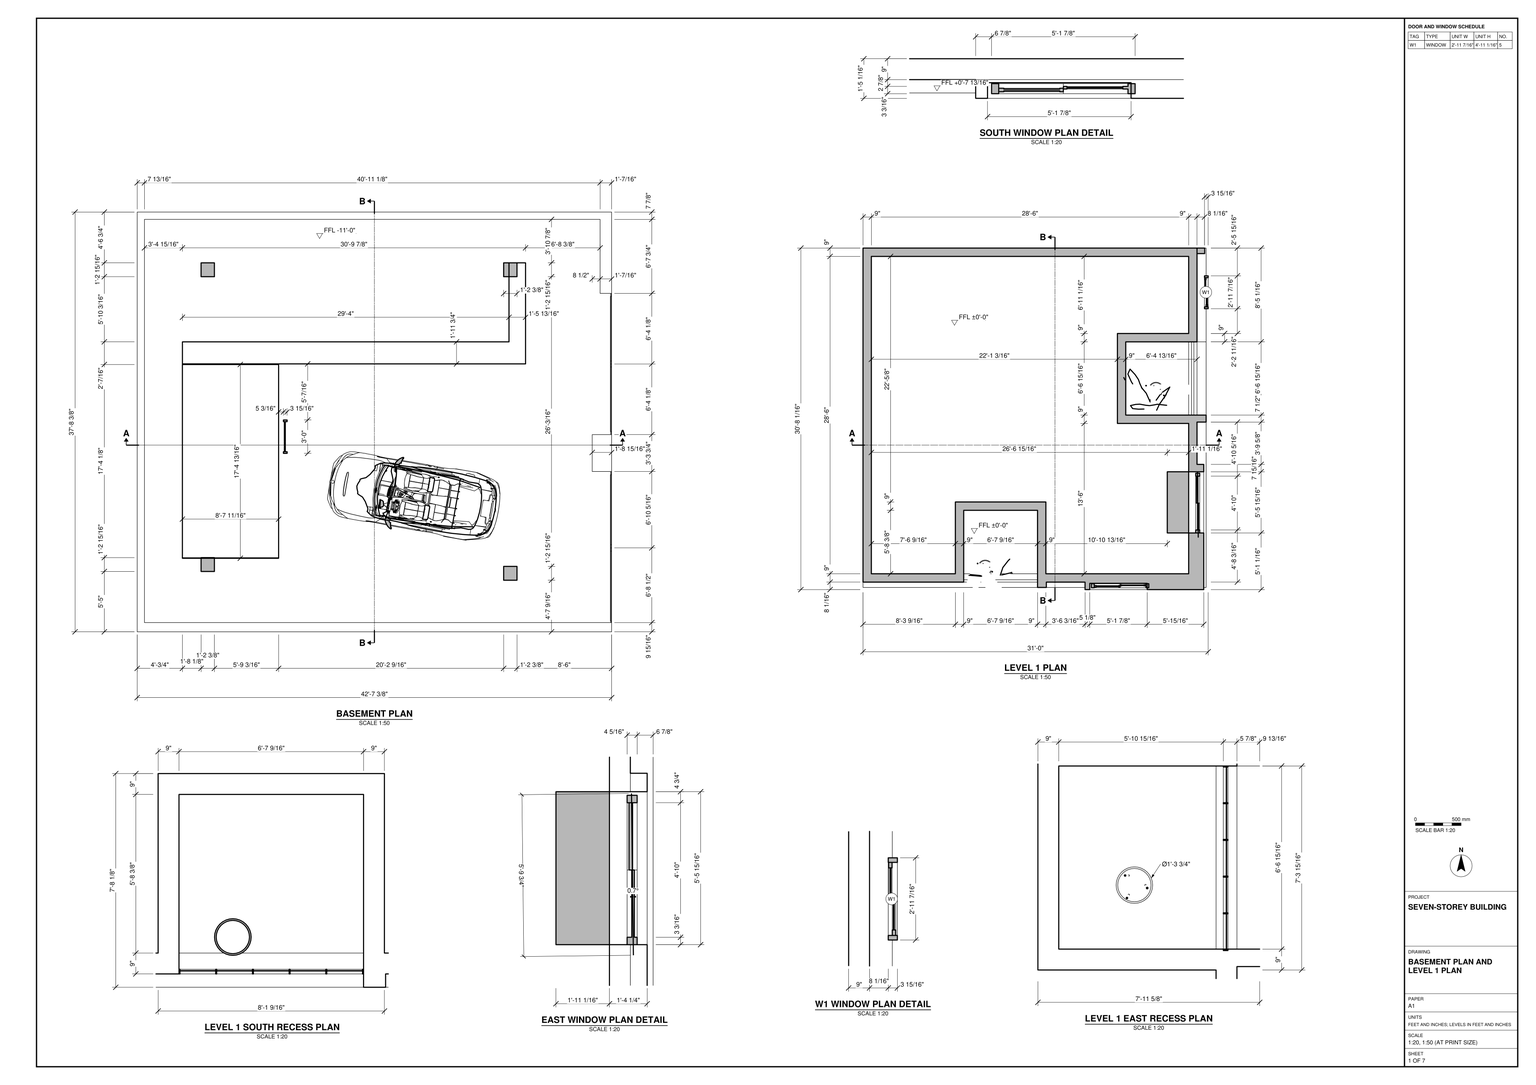
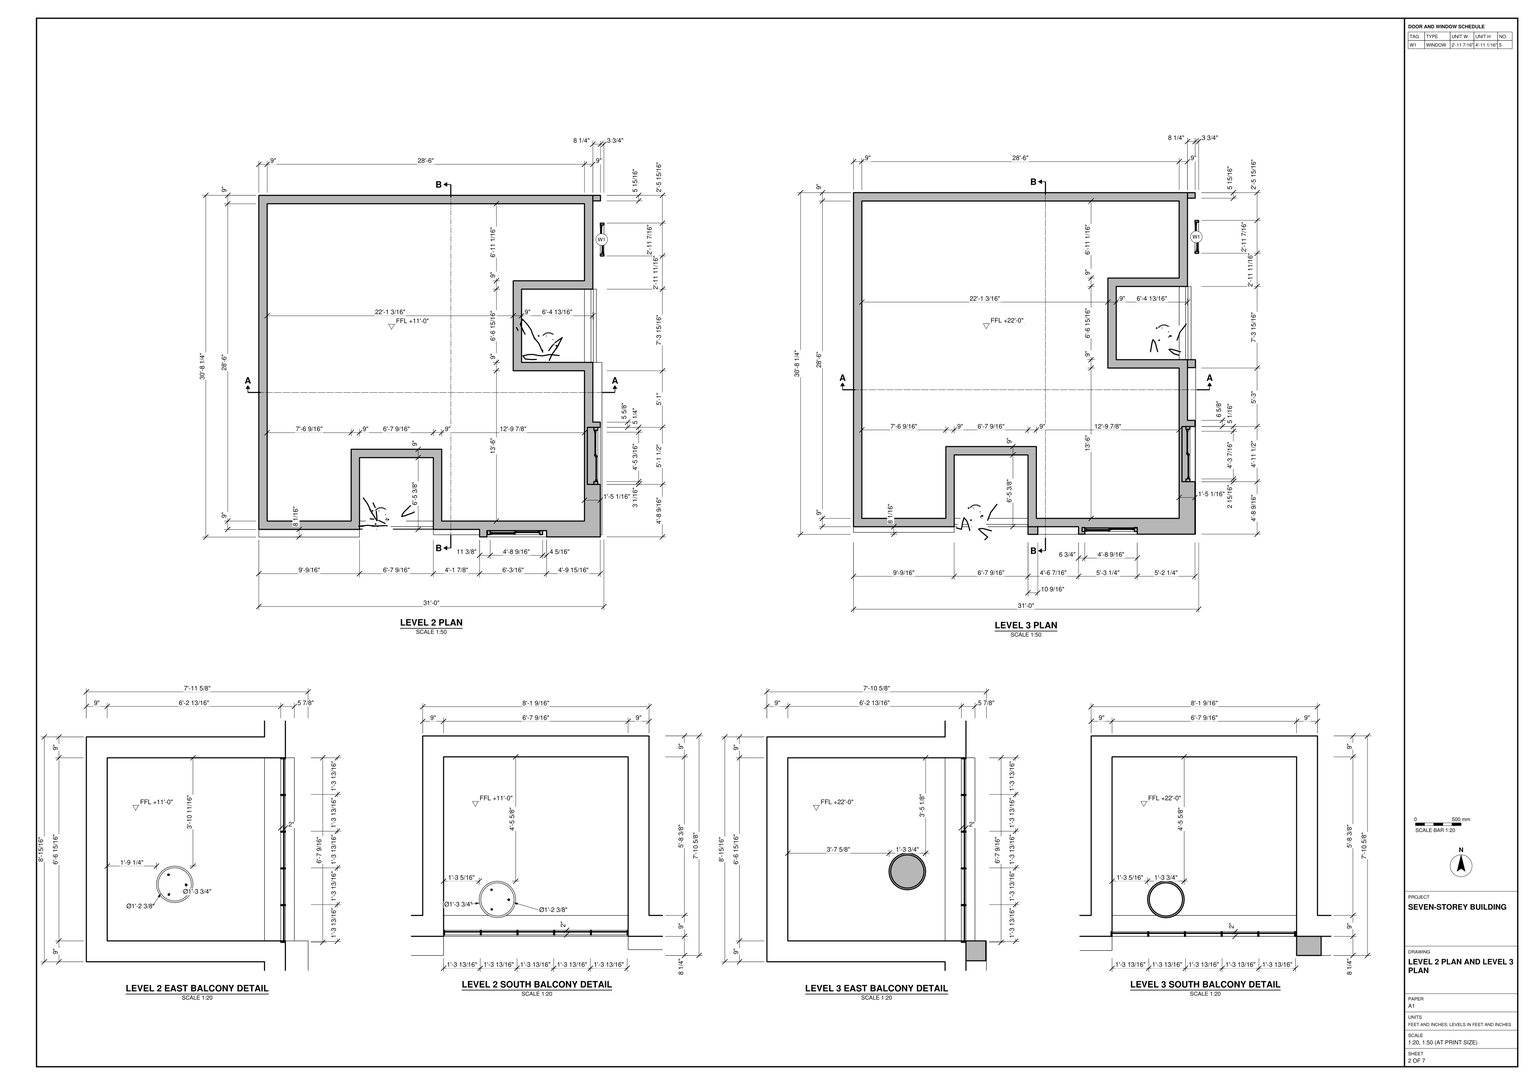
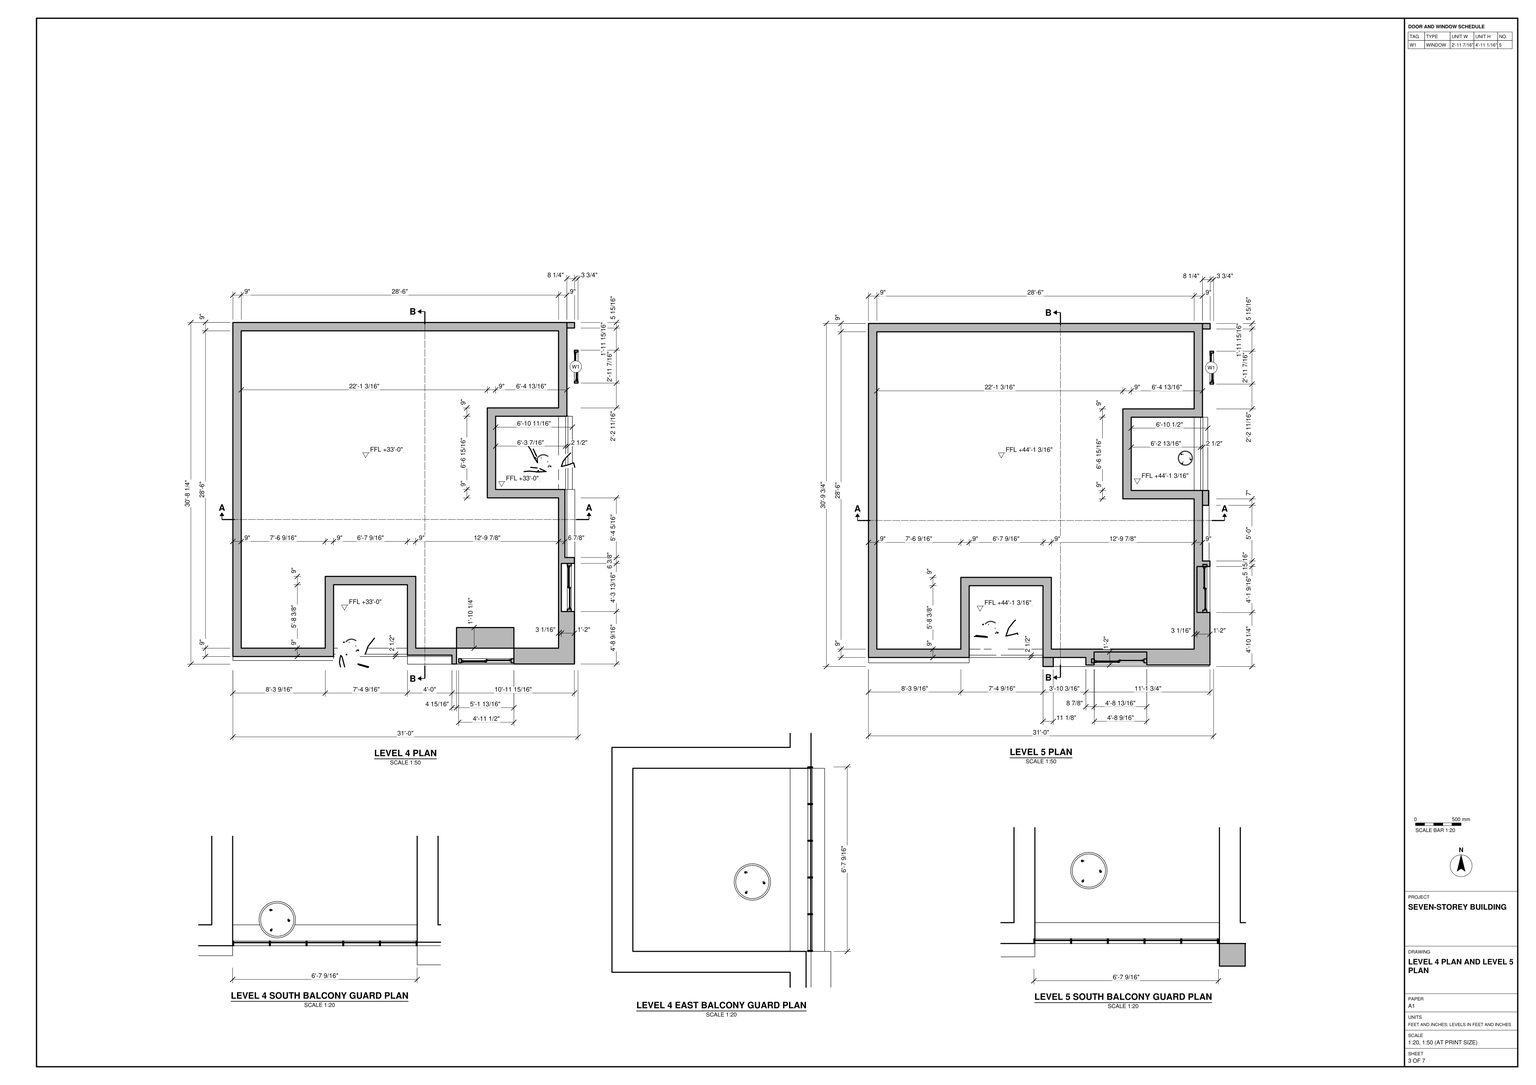
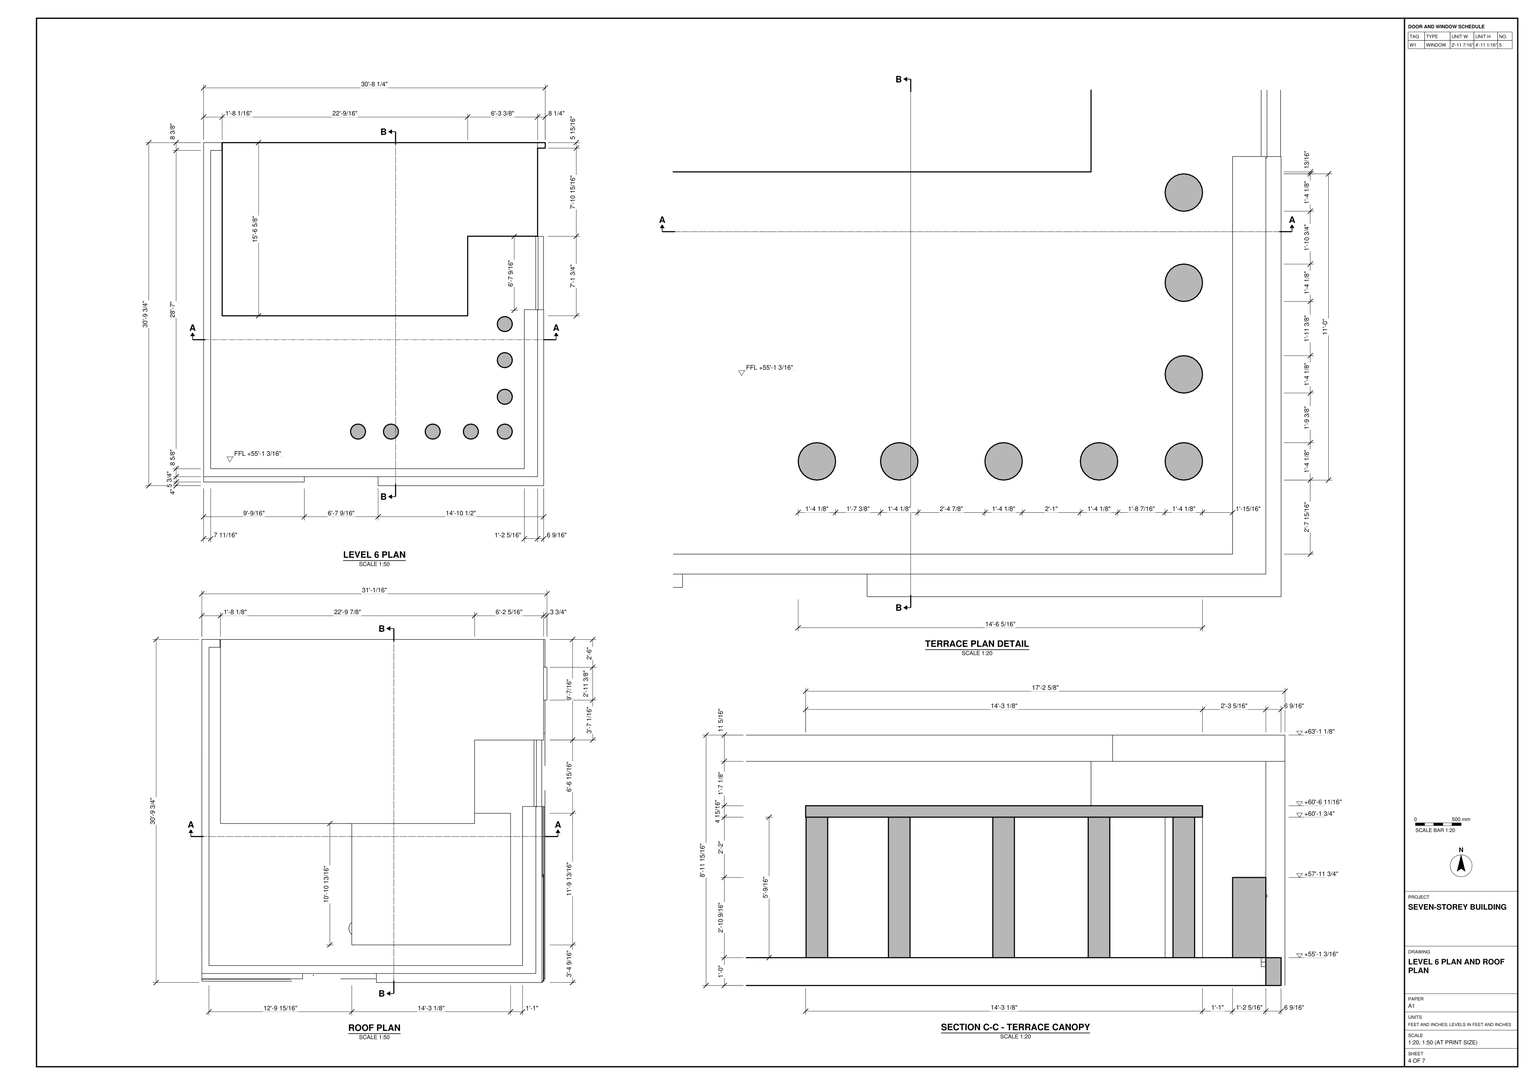
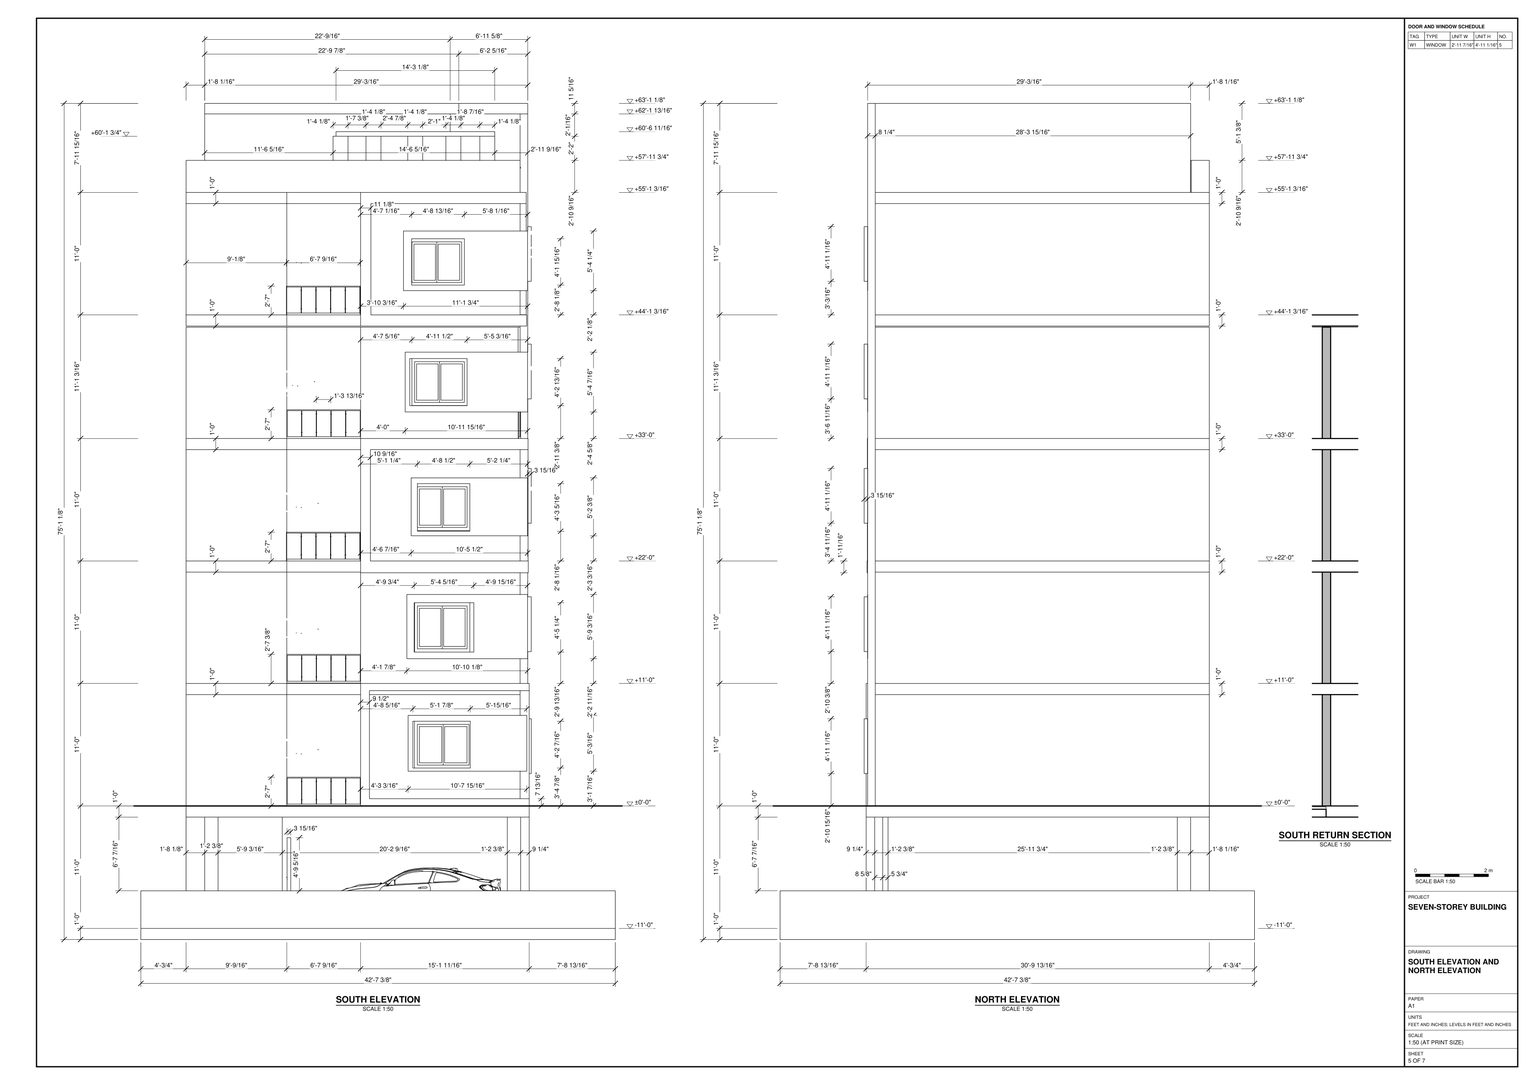
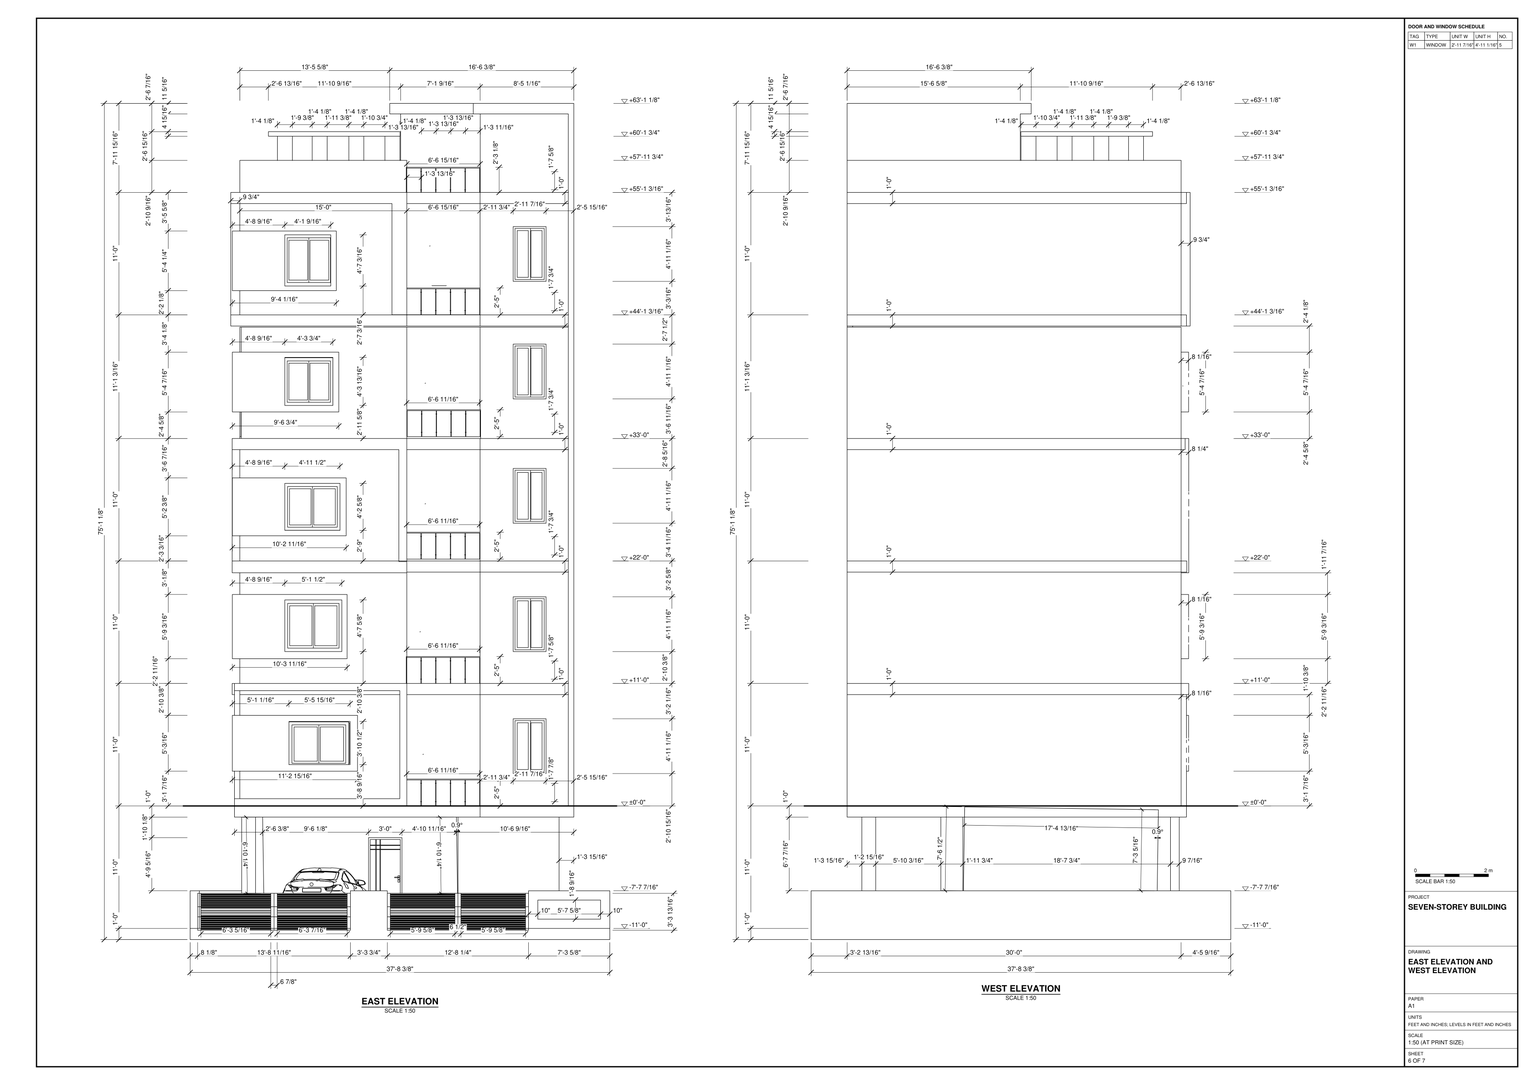
Build the seven-storey building in SketchUp from task_files/diagram_01.pdf. Work in feet and inches. The overall model measures 42'-7 3/8" along X, 37'-8 3/8" along Y and 75'-1 1/8" along Z. Set the floor levels, relative to the ground floor, at -11'-0", ±0'-0", +11'-0", +22'-0", +33'-0", +44'-1 3/16" and +55'-1 3/16".

Start with the wider basement footprint. Follow its perimeter, square supports and stepped internal outline, leaving the parking area open for the vehicle shown in plan. Above it, build the floor slabs and perimeter walls. Use the 9" wall thickness where marked and follow the local changes in thickness at the window bays. Set the south and east bays back into the floor plate to form the ground-floor recesses and upper balconies. Use the enlarged plans to locate the guards at the open edges and the planters behind them. Place the window units according to each floor plan rather than assuming all openings align. Complete the roof and its edges as drawn.

Keep walls, slabs, roof elements and each furniture or joinery piece in separate groups or components, and use components for repeated parts. Decor and loose items, including planters and the parked vehicle, may be any suitable library components. Save one SketchUp model as output_files/building_with_basement_parking_and_recessed_balconies.skp.

# SketchUp Ruby script. Lengths in inches.
U = 1.inch
M = Sketchup.active_model
def pt(a) = Geom::Point3d.new(a.map { |v| v * U })
def face(e, loops, mat)
  f = e.add_face(loops[0].map { |a| pt(a) })
  loops[1..].each { |l| e.add_face(l.map { |a| pt(a) }).erase! }
  f.material = f.back_material = mat if mat
  f
end
# faces: each face lists its corners as indices into pts; further lists are holes
def faces(e, pts, list, mat = nil) = list.each { |f| face(e, (f[0].is_a?(Array) ? f : [f]).map { |l| l.map { |i| pts[i] } }, mat) }
# xy, xz, yz: faces in a plane at the given z, y or x. An outline is a flat list of corners, or four numbers for a rectangle; further outlines are holes
def ring(l) = l.size == 4 ? [[l[0], l[1]], [l[2], l[1]], [l[2], l[3]], [l[0], l[3]]] : l.each_slice(2).to_a
def flat(e, list, mat, &to3) = list.each { |f| face(e, (f[0].is_a?(Array) ? f : [f]).map { |l| ring(l).map { |u, v| to3.(u, v) } }, mat) }
def xy(e, z, list, mat = nil) = flat(e, list, mat) { |x, y| [x, y, z] }
def xz(e, y, list, mat = nil) = flat(e, list, mat) { |x, z| [x, y, z] }
def yz(e, x, list, mat = nil) = flat(e, list, mat) { |y, z| [x, y, z] }
def lines(e, pts, list) = list.each { |a, b| e.add_line(pt(pts[a]), pt(pts[b])) }
# prism: a flat outline (further loops are holes) pulled along v
def prism(e, loops, v, mat = nil)
  f = face(e, loops, mat); d = Geom::Vector3d.new(v.map { |x| x * U })
  f.pushpull(f.normal.samedirection?(d) ? d.length : -d.length)
end
def box(e, o, s, mat = nil) = prism(e, [[o, [o[0] + s[0], o[1], o[2]], [o[0] + s[0], o[1] + s[1], o[2]], [o[0], o[1] + s[1], o[2]]]], [0, 0, s[2]], mat)
def at(x, y, z, deg = 0) = Geom::Transformation.translation(pt([x, y, z])) * Geom::Transformation.rotation(ORIGIN, Z_AXIS, deg.degrees)
def axes(o, x, y, z) = Geom::Transformation.new([*x, 0, *y, 0, *z, 0, *pt(o).to_a, 1])
def part(name) = M.definitions.add(name)
# library, detail: a bought-in or finely detailed component or shape, given as its bounding box
def library(name, o, s) = part(name).tap { |d| box(d.entities, o, s) }
def detail(e, o, s) = box(e.add_group.entities, o, s)
def put(e, d, t, mat = nil) = e.add_instance(d, t).tap { |i| i.material = mat if mat }
def group(e, t, mat = nil) = e.add_group.tap { |g| g.transformation = t; g.material = mat if mat }.entities
root = M.entities
M.materials.add("[Color M00]").color = [255, 255, 255]
M.materials.add("[Wood Veneer 01]").color = [120, 70, 37]
M.materials.add("[Wood Veneer 02]").color = [190, 128, 91]
c1 = library("Sliding window\#1",[0,0,0],[4.33,55.51,41.34])
c2 = library("Sliding Window",[0,0,0],[35.43,4.93,59.06])
c3 = library("Ver Glass Railing",[0,0,0],[2.5,185,31])
c4 = library("Round Planter with Plant",[-35.48,-39.77,0],[80.62,63.55,77.875])
c5 = library("Porton casa",[225.62,-50.57,0],[86.62,1.75,86.61])
c6 = library("Untitled",[0,0,0],[36,4.39,84])
c7 = library("002 Bmw M4 + mat3.4 2017",[-252.8,19.48,9.01],[196.94,171.32,55.15])
c8 = part("Group\#3")
box(c8.entities,[0,-360,0],[360,360,12])
c9 = part("Group\#4")
box(c9.entities,[0,0,-120],[14.375,14.9375,120])
c10 = library("Group\#5",[0,0,0],[16.125,16.125,60.5625])
xy(root,-144,[[0,0,79.875,276.3125],[79.875,0,511.375,276.3125],[0,276.3125,79.875,452.375],[79.875,276.3125,511.375,452.375]])
xy(root,-132,[[7.83,9.96,511.375,9.96,511.375,172.78,490.4375,172.78,490.4375,212.53,511.375,212.53,511.375,364.75,498.9375,364.75,498.9375,444.5,7.83,444.5]])
xy(root,-128.875,[[48.78,288.75,48.78,312.5,400.75,312.5,400.75,397.65,418.59,397.65,418.59,288.75]])
xy(root,-122,[[508.4375,374.75,511.375,442.38]],"[Wood Veneer 01]")
xy(root,-101.43,[[508.4375,374.75,511.375,442.38]],"[Wood Veneer 01]")
xy(root,-91.4375,[[0,0,511.375,0,511.375,9.96,7.83,9.96,7.83,444.5,498.9375,444.5,498.9375,364.75,511.375,364.75,511.375,452.375,0,452.375],[490.4375,172.78,511.375,212.53]])
xy(root,-12,[[48.78,288.75,418.59,288.75,418.59,397.65,400.75,397.65,400.75,312.5,48.78,312.5]])
xy(root,0,[[[236.875,47.8125,418.59,47.8125,418.59,233.5625,331.96,233.5625,331.96,312.5,408.78,312.5,408.78,413.5625,48.78,413.5625,48.78,53.5625,157.3125,53.5625,157.3125,130.9375,236.875,130.9375],[57.78,62.5625,57.78,404.5625,399.78,404.5625,399.78,321.5,322.96,321.5,322.96,224.5625,399.78,224.5625,399.78,62.5625,245.875,62.5625,245.875,139.9375,148.3125,139.9375,148.3125,62.5625]],[157.3125,53.5625,236.875,62.5625],[57.78,62.5625,148.3125,62.5625,148.3125,139.9375,245.875,139.9375,245.875,62.5625,399.78,62.5625,399.78,224.5625,322.96,224.5625,322.96,321.5,399.78,321.5,399.78,404.5625,57.78,404.5625],[157.3125,62.5625,236.875,130.9375],[331.96,233.5625,399.78,312.5],
  [399.78,233.5625,408.78,312.5],[408.78,407.61,417.03,413.5625]])
xy(root,7.82,[[246.39,47.8125,418.59,47.8125,418.59,226.03,408.78,226.03,408.78,53.5625,246.39,53.5625]])
xy(root,37.42,[[288.09,45.5,288.09,53.5625,408.78,53.5625,408.78,180.43,416.03,180.43,416.03,45.5]])
xy(root,40.86,[[293.2,45.5,355.07,52.25]])
xy(root,44.57,[[376.71,106.54,416.03,172.48]])
xy(root,91.07,[[376.71,106.54,416.03,172.48]])
xy(root,91.3,[[293.2,45.5,355.07,52.25]])
xy(root,97.61,[[288.09,45.5,416.03,45.5,416.03,180.43,408.78,180.43,408.78,53.5625,288.09,53.5625]])
xy(root,120,[[331.96,233.5625,412.65,312.5]])
xy(root,120,[[48.78,45.3125,157.3125,53.5625]],"[Wood Veneer 01]")
xy(root,124.25,[[246.39,47.8125,246.39,53.5625,408.78,53.5625,408.78,226.03,418.59,226.03,418.59,47.8125]])
xy(root,132,[[236.875,47.8125,418.59,47.8125,418.59,233.5625,408.78,233.5625,408.78,53.5625,236.875,53.5625],[[48.78,53.5625,157.3125,53.5625,157.3125,130.9375,236.875,130.9375,236.875,53.5625,408.78,53.5625,408.78,233.5625,331.96,233.5625,331.96,312.5,408.78,312.5,408.78,413.5625,48.78,413.5625],[57.78,62.5625,57.78,404.5625,399.78,404.5625,399.78,321.5,322.96,321.5,322.96,224.5625,399.78,224.5625,399.78,62.5625,245.875,62.5625,245.875,139.9375,148.3125,139.9375,148.3125,62.5625]],[157.3125,53.5625,236.875,62.5625],[57.78,62.5625,148.3125,62.5625,148.3125,139.9375,245.875,139.9375,245.875,62.5625,399.78,62.5625,399.78,224.5625,322.96,224.5625,322.96,321.5,399.78,321.5,399.78,404.5625,57.78,404.5625],[157.3125,62.5625,236.875,130.9375],
  [331.96,233.5625,399.78,312.5],[399.78,233.5625,412.65,312.5]])
xy(root,132,[[48.78,45.3125,157.3125,53.5625]],"[Wood Veneer 01]")
xy(root,158.68,[[286.72,45.5,286.72,53.5625,408.78,53.5625,408.78,169.1875,416.84,169.1875,416.84,45.5]])
xy(root,165.8,[[294.61,45.5,358.92,52.25]])
xy(root,166.38,[[402.84,102.07,416.84,163.54]])
xy(root,219.05,[[294.61,45.5,358.92,52.25]])
xy(root,222.02,[[402.84,102.07,416.84,163.54]])
xy(root,227.89,[[286.72,45.5,416.84,45.5,416.84,169.1875,408.78,169.1875,408.78,53.5625,286.72,53.5625]])
xy(root,251.3125,[[236.875,45.3125,236.875,53.5625,408.78,53.5625,408.78,233.5625,417.59,233.5625,417.59,45.3125]])
xy(root,252,[[[48.78,53.5625,157.3125,53.5625,157.3125,130.9375,236.875,130.9375,236.875,53.5625,408.78,53.5625,408.78,233.5625,331.96,233.5625,331.96,312.5,408.78,312.5,408.78,413.5625,48.78,413.5625],[57.78,62.5625,57.78,404.5625,399.78,404.5625,399.78,321.5,322.96,321.5,322.96,224.5625,399.78,224.5625,399.78,62.5625,245.875,62.5625,245.875,139.9375,148.3125,139.9375,148.3125,62.5625]],[331.96,233.5625,412.65,312.5]])
xy(root,252,[[48.78,47.4375,157.3125,53.5625]],"[Wood Veneer 01]")
xy(root,263.3125,[[408.78,225,417.34,233.5625]])
xy(root,264,[[247.45,45.3125,417.59,45.3125,417.59,233.5625,408.78,233.5625,408.78,53.5625,247.45,53.5625],[[48.78,53.5625,157.3125,53.5625,157.3125,130.9375,236.875,130.9375,236.875,53.5625,408.78,53.5625,408.78,233.5625,331.96,233.5625,331.96,312.5,408.78,312.5,408.78,413.5625,48.78,413.5625],[57.78,62.5625,57.78,404.5625,399.78,404.5625,399.78,321.5,322.96,321.5,322.96,224.5625,399.78,224.5625,399.78,62.5625,245.875,62.5625,245.875,139.9375,148.3125,139.9375,148.3125,62.5625]],[157.3125,53.5625,236.875,62.5625],[57.78,62.5625,148.3125,62.5625,148.3125,139.9375,245.875,139.9375,245.875,62.5625,399.78,62.5625,399.78,224.5625,322.96,224.5625,322.96,321.5,399.78,321.5,399.78,404.5625,57.78,404.5625],[157.3125,62.5625,236.875,130.9375],
  [331.96,233.5625,399.78,312.5],[399.78,233.5625,412.65,312.5]])
xy(root,264,[[48.78,47.4375,157.3125,53.5625]],"[Wood Veneer 01]")
xy(root,291.16,[[291.34,45.5,291.34,53.5625,408.78,53.5625,408.78,168.1875,416.84,168.1875,416.84,45.5]])
xy(root,296.08,[[298.12,45.5,354.62,52.25]])
xy(root,297.09,[[402.84,102.07,416.84,161.55]])
xy(root,347.39,[[298.12,45.5,354.62,52.25]])
xy(root,347.65,[[402.84,102.07,416.84,161.55]])
xy(root,353.54,[[291.34,45.5,416.84,45.5,416.84,168.1875,408.78,168.1875,408.78,53.5625,291.34,53.5625]])
xy(root,384,[[247.45,45.3125,247.45,53.5625,408.78,53.5625,408.78,225,417.34,225,417.34,45.3125],[[48.78,53.5625,157.3125,53.5625,157.3125,130.9375,236.875,130.9375,236.875,53.5625,408.78,53.5625,408.78,233.5625,331.96,233.5625,331.96,312.5,408.78,312.5,408.78,413.5625,48.78,413.5625],[57.78,62.5625,57.78,404.5625,399.78,404.5625,399.78,321.5,322.96,321.5,322.96,224.5625,399.78,224.5625,399.78,62.5625,245.875,62.5625,245.875,139.9375,148.3125,139.9375,148.3125,62.5625]],[331.96,233.5625,414.65,312.5]])
xy(root,384,[[48.78,49.25,157.3125,53.5625]],"[Wood Veneer 01]")
xy(root,396,[[236.875,45.3125,417.34,45.3125,417.34,233.5625,408.78,233.5625,408.78,53.5625,236.875,53.5625],[[48.78,53.5625,157.3125,53.5625,157.3125,130.9375,236.875,130.9375,236.875,55.0625,406.65,55.0625,406.65,233.5625,331.96,233.5625,331.96,312.5,408.78,312.5,408.78,413.5625,48.78,413.5625],[57.78,62.5625,57.78,404.5625,399.78,404.5625,399.78,321.5,322.96,321.5,322.96,224.5625,399.78,224.5625,399.78,62.5625,245.875,62.5625,245.875,139.9375,148.3125,139.9375,148.3125,62.5625]],[157.3125,53.5625,236.875,62.5625],[236.875,53.5625,408.78,55.0625],[406.65,55.0625,408.78,233.5625],
  [57.78,62.5625,148.3125,62.5625,148.3125,139.9375,245.875,139.9375,245.875,62.5625,399.78,62.5625,399.78,224.5625,322.96,224.5625,322.96,321.5,399.78,321.5,399.78,404.5625,57.78,404.5625],[157.3125,62.5625,236.875,130.9375],[331.96,233.5625,399.78,312.5],[399.78,233.5625,414.65,312.5]])
xy(root,396,[[48.78,49.25,157.3125,53.5625]],"[Wood Veneer 01]")
xy(root,424.61,[[284.9,45.5,284.9,55.0625,406.65,55.0625,406.65,160.25,416.84,160.25,416.84,45.5]])
xy(root,431.34,[[289.83,45.5,351.64,84.8125]])
xy(root,431.59,[[402.84,102.07,416.84,153.88]])
xy(root,482.16,[[289.83,45.5,351.64,84.8125]])
xy(root,483.41,[[402.84,102.07,416.84,153.88]])
xy(root,489.05,[[284.9,45.5,416.84,45.5,416.84,160.25,406.65,160.25,406.65,55.0625,284.9,55.0625]])
xy(root,516,[[[48.78,53.5625,157.3125,53.5625,157.3125,130.9375,236.875,130.9375,236.875,55.0625,406.65,55.0625,406.65,233.5625,331.96,233.5625,331.96,312.5,408.78,312.5,408.78,413.5625,48.78,413.5625],[57.78,62.5625,57.78,404.5625,399.78,404.5625,399.78,321.5,322.96,321.5,322.96,224.5625,399.78,224.5625,399.78,62.5625,245.875,62.5625,245.875,139.9375,148.3125,139.9375,148.3125,62.5625]]])
xy(root,517.1875,[[236.875,43.8125,236.875,53.5625,408.78,53.5625,408.78,233.5625,415.9,233.5625,415.9,43.8125],[408.78,233.5625,414.46,312.47]])
xy(root,517.1875,[[48.78,47.8125,157.3125,53.5625]],"[Wood Veneer 01]")
xy(root,529.1875,[[247.98,43.8125,415.9,43.8125,415.9,233.5625,408.78,233.5625,408.78,53.5625,247.98,53.5625],[[48.78,53.5625,157.3125,53.5625,157.3125,130.9375,236.875,130.9375,236.875,53.5625,408.78,53.5625,408.78,233.5625,331.96,233.5625,331.96,312.5,408.78,312.5,408.78,413.5625,48.78,413.5625],[57.78,62.5625,57.78,404.5625,399.78,404.5625,399.78,321.5,322.96,321.5,322.96,224.5625,399.78,224.5625,399.78,62.5625,245.875,62.5625,245.875,139.9375,148.3125,139.9375,148.3125,62.5625]],[157.3125,53.5625,236.875,62.5625],[57.78,62.5625,148.3125,62.5625,148.3125,139.9375,245.875,139.9375,245.875,62.5625,399.78,62.5625,399.78,224.5625,322.96,224.5625,322.96,321.5,399.78,321.5,399.78,404.5625,57.78,404.5625],[157.3125,62.5625,236.875,130.9375],
  [331.96,233.5625,399.78,312.5],[399.78,233.5625,408.78,312.5],[408.78,233.5625,414.46,312.47]])
xy(root,529.1875,[[48.78,47.8125,157.3125,53.5625]],"[Wood Veneer 01]")
xy(root,529.375,[[408.78,217.55,415.36,233.5625]])
xy(root,555.34,[[283.09,45.5,283.09,53.5625,408.78,53.5625,408.78,157.5625,416.84,157.5625,416.84,45.5]])
xy(root,560.35,[[402.84,102.07,416.84,151.63]])
xy(root,561.34,[[291.94,45.5,348.75,59.5]])
xy(root,611.28,[[291.94,45.5,348.75,59.5]])
xy(root,615.53,[[402.84,102.07,416.84,151.63]])
xy(root,619.59,[[283.09,45.5,416.84,45.5,416.84,157.5625,408.78,157.5625,408.78,53.5625,283.09,53.5625]])
xy(root,649.1875,[[247.98,43.8125,247.98,53.5625,408.78,53.5625,408.78,217.55,415.36,217.55,415.36,43.8125],[[48.78,53.5625,157.3125,53.5625,157.3125,130.9375,236.875,130.9375,236.875,53.5625,408.78,53.5625,408.78,233.5625,331.96,233.5625,331.96,312.5,408.78,312.5,408.78,413.5625,48.78,413.5625],[57.78,62.5625,57.78,404.5625,399.78,404.5625,399.78,321.5,322.96,321.5,322.96,224.5625,399.78,224.5625,399.78,62.5625,245.875,62.5625,245.875,139.9375,148.3125,139.9375,148.3125,62.5625]],[331.96,233.5625,415.15,312.5]])
xy(root,649.1875,[[48.78,47.8125,157.3125,53.5625]],"[Wood Veneer 01]")
xy(root,661.1875,[[236.875,43.8125,415.36,43.8125,415.36,233.5625,408.78,233.5625,408.78,53.5625,236.875,53.5625],[48.78,53.5625,48.78,413.5625,68.34,413.5625,68.34,405.16,56.47,405.16,56.47,62.16,394.46,62.16,394.46,233.5625,408.78,233.5625,408.78,53.5625],[68.84,226.9375,68.84,413.5625,408.78,413.5625,408.78,312.6875,333.43,312.6875,333.43,226.9375],[408.78,233.5625,415.15,312.5]])
xy(root,661.1875,[[48.78,47.8125,157.3125,53.5625]],"[Wood Veneer 01]")
xy(root,695.75,[[48.78,53.5625,408.78,53.5625,408.78,233.5625,394.46,233.5625,394.46,62.16,56.47,62.16,56.47,405.16,68.34,405.16,68.34,413.5625,48.78,413.5625]])
xy(root,745.81,[[68.84,215.1875,68.84,226.9375,333.43,226.9375,333.43,312.6875,408.78,312.6875,408.78,407.61,417.03,407.61,417.03,305.15,342.74,305.15,342.74,215.1875]],"[Wood Veneer 01]")
xy(root,757.125,[[68.84,215.1875,342.74,215.1875,342.74,305.15,417.03,305.15,417.03,413.5625,68.84,413.5625]])
xz(root,0,[[0,-144,511.375,-132],[0,-132,511.375,-91.4375]])
xz(root,9.96,[[7.83,-132,511.375,-91.4375]])
xz(root,43.8125,[[236.875,517.1875,415.9,517.1875,415.9,529.1875,247.98,529.1875,247.98,649.1875,415.36,649.1875,415.36,661.1875,236.875,661.1875]])
xz(root,45.3125,[[236.875,251.3125,417.59,251.3125,417.59,264,247.45,264,247.45,384,417.34,384,417.34,396,236.875,396]])
xz(root,45.3125,[[48.78,120,157.3125,132]],"[Wood Veneer 01]")
xz(root,45.5,[[[288.09,37.42,416.03,97.61],[293.2,40.86,355.07,91.3]],[[286.72,158.68,416.84,227.89],[294.61,165.8,358.92,219.05]],[[291.34,291.16,416.84,353.54],[298.12,296.08,354.62,347.39]],[[284.9,424.61,416.84,489.05],[289.83,431.34,351.64,482.16]],[[283.09,555.34,416.84,619.59],[291.94,561.34,348.75,611.28]]])
xz(root,47.4375,[[48.78,252,157.3125,264]],"[Wood Veneer 01]")
xz(root,47.8125,[[236.875,0,418.59,0,418.59,7.82,246.39,7.82,246.39,124.25,418.59,124.25,418.59,132,236.875,132]])
xz(root,47.8125,[[48.78,517.1875,157.3125,529.1875],[48.78,649.1875,157.3125,661.1875]],"[Wood Veneer 01]")
xz(root,49.25,[[48.78,384,157.3125,396]],"[Wood Veneer 01]")
xz(root,52.25,[[293.2,40.86,355.07,91.3],[294.61,165.8,358.92,219.05],[298.12,296.08,354.62,347.39]])
xz(root,53.5625,[[48.78,0,157.3125,120],[236.875,120,236.875,132,408.78,132,408.78,124.25,246.39,124.25,246.39,120],[246.39,120,408.78,124.25],[48.78,132,157.3125,252],[236.875,132,408.78,132,408.78,158.68,286.72,158.68,286.72,227.89,408.78,227.89,408.78,251.3125,236.875,251.3125],
  [236.875,251.3125,408.78,252],[236.875,252,408.78,264],[48.78,264,157.3125,384],[236.875,264,247.45,384],[236.875,384,408.78,396],
  [48.78,396,157.3125,516],[48.78,517.1875,157.3125,529.1875],[236.875,517.1875,408.78,529.1875],[48.78,529.1875,157.3125,649.1875],[236.875,649.1875,408.78,661.1875],
  [48.78,661.1875,408.78,695.75]])
xz(root,53.5625,[[246.39,7.82,408.78,7.82,408.78,37.42,288.09,37.42,288.09,97.61,408.78,97.61,408.78,120,246.39,120],[247.45,264,408.78,264,408.78,291.16,291.34,291.16,291.34,353.54,408.78,353.54,408.78,384,247.45,384],[236.875,529.1875,247.98,649.1875],[247.98,529.1875,408.78,529.1875,408.78,555.34,283.09,555.34,283.09,619.59,408.78,619.59,408.78,649.1875,247.98,649.1875]],"[Wood Veneer 02]")
xz(root,55.0625,[[236.875,396,406.65,396,406.65,424.61,284.9,424.61,284.9,489.05,406.65,489.05,406.65,516,236.875,516]])
xz(root,59.5,[[291.94,561.34,348.75,611.28]])
xz(root,62.16,[[56.47,661.1875,394.46,695.75]])
xz(root,62.5625,[[57.78,0,148.3125,120],[245.875,0,399.78,120],[57.78,132,148.3125,252],[245.875,132,399.78,252],[57.78,264,148.3125,384],
  [245.875,264,399.78,384],[57.78,396,148.3125,516],[57.78,529.1875,148.3125,649.1875],[245.875,529.1875,399.78,649.1875]])
xz(root,62.5625,[[245.875,396,399.78,516]],"[Color M00]")
xz(root,84.8125,[[289.83,431.34,351.64,482.16]])
xz(root,102.07,[[402.84,166.38,416.84,222.02],[402.84,297.09,416.84,347.65],[402.84,431.59,416.84,483.41],[402.84,560.35,416.84,615.53]])
xz(root,106.54,[[376.71,44.57,416.03,91.07]])
xz(root,130.9375,[[157.3125,0,236.875,120],[157.3125,132,236.875,252],[157.3125,264,236.875,384],[157.3125,396,236.875,516],[157.3125,529.1875,236.875,649.1875]])
xz(root,139.9375,[[148.3125,0,245.875,120],[148.3125,132,245.875,252],[148.3125,264,245.875,384],[148.3125,396,245.875,516],[148.3125,529.1875,245.875,649.1875]])
xz(root,151.63,[[402.84,560.35,416.84,615.53]])
xz(root,153.88,[[402.84,431.59,416.84,483.41]])
xz(root,157.5625,[[408.78,555.34,416.84,619.59]])
xz(root,160.25,[[406.65,424.61,416.84,489.05]])
xz(root,161.55,[[402.84,297.09,416.84,347.65]])
xz(root,163.54,[[402.84,166.38,416.84,222.02]])
xz(root,168.1875,[[408.78,291.16,416.84,353.54]])
xz(root,169.1875,[[408.78,158.68,416.84,227.89]])
xz(root,172.48,[[376.71,44.57,416.03,91.07]])
xz(root,172.78,[[490.4375,-132,511.375,-91.4375]])
xz(root,180.43,[[408.78,37.42,416.03,97.61]])
xz(root,212.53,[[490.4375,-132,511.375,-91.4375]])
xz(root,215.1875,[[68.84,745.81,342.74,757.125]],"[Wood Veneer 01]")
xz(root,217.55,[[408.78,529.375,415.36,649.1875]])
xz(root,224.5625,[[322.96,0,399.78,120],[322.96,132,399.78,252],[322.96,264,399.78,384],[322.96,396,399.78,516],[322.96,529.1875,399.78,649.1875]])
xz(root,225,[[408.78,263.3125,417.34,384]])
xz(root,226.03,[[408.78,7.82,418.59,124.25]])
xz(root,226.9375,[[68.84,661.1875,333.43,745.81]])
xz(root,233.5625,[[331.96,0,399.78,120],[399.78,0,408.78,120],[408.78,0,408.78,120,412.65,120,412.65,132,418.59,132,418.59,0],[408.78,120,412.65,132],[331.96,132,399.78,252],
  [399.78,132,408.78,252],[408.78,251.3125,408.78,252,412.65,252,412.65,263.3125,417.34,263.3125,417.34,264,417.59,264,417.59,251.3125],[408.78,252,412.65,263.3125],[408.78,263.3125,412.65,264],[412.65,263.3125,417.34,264],
  [331.96,264,399.78,384],[399.78,264,408.78,384],[408.78,264,408.78,384,414.65,384,414.65,396,417.34,396,417.34,264],[408.78,384,414.65,396],[331.96,396,399.78,516],
  [399.78,396,406.65,516],[408.78,517.1875,414.46,529.1875],[414.46,517.1875,415.9,529.1875],[331.96,529.1875,399.78,649.1875],[399.78,529.1875,408.78,649.1875],
  [408.78,529.375,408.78,649.1875,415.15,649.1875,415.15,661.1875,415.36,661.1875,415.36,529.375],[408.78,649.1875,415.15,661.1875],[394.46,661.1875,408.78,695.75]])
xz(root,288.75,[[48.78,-128.875,418.59,-12]])
xz(root,305.15,[[342.74,745.81,417.03,757.125]],"[Wood Veneer 01]")
xz(root,312.47,[[408.78,517.1875,414.46,529.1875]])
xz(root,312.5,[[48.78,-128.875,400.75,-12],[331.96,0,399.78,120],[399.78,0,408.78,120],[408.78,120,412.65,132],[331.96,132,399.78,252],
  [399.78,132,408.78,252],[408.78,252,412.65,264],[331.96,264,399.78,384],[399.78,264,408.78,384],[408.78,384,414.65,396],
  [331.96,396,399.78,516],[399.78,396,408.78,516],[331.96,529.1875,399.78,649.1875],[399.78,529.1875,408.78,649.1875],[408.78,649.1875,415.15,661.1875]])
xz(root,312.6875,[[333.43,661.1875,408.78,745.81]])
xz(root,321.5,[[322.96,0,399.78,120],[322.96,132,399.78,252],[322.96,264,399.78,384],[322.96,396,399.78,516],[322.96,529.1875,399.78,649.1875]])
xz(root,364.75,[[498.9375,-132,511.375,-91.4375]])
xz(root,374.75,[[508.4375,-122,511.375,-101.43]],"[Wood Veneer 01]")
xz(root,397.65,[[400.75,-128.875,418.59,-12]])
xz(root,404.5625,[[57.78,0,399.78,120],[57.78,132,399.78,252],[57.78,264,399.78,384],[57.78,396,399.78,516],[57.78,529.1875,399.78,649.1875]])
xz(root,405.16,[[56.47,661.1875,68.34,695.75]])
xz(root,407.61,[[408.78,0,417.03,745.81]],"[Wood Veneer 01]")
xz(root,413.5625,[[48.78,0,408.78,120],[48.78,132,408.78,252],[48.78,264,408.78,384],[48.78,396,408.78,516],[48.78,529.1875,408.78,649.1875],
  [48.78,661.1875,68.34,695.75],[68.84,661.1875,408.78,757.125]])
xz(root,413.5625,[[408.78,0,417.03,757.125]],"[Wood Veneer 01]")
xz(root,442.38,[[508.4375,-122,511.375,-101.43]],"[Wood Veneer 01]")
xz(root,444.5,[[7.83,-132,498.9375,-91.4375]])
xz(root,452.375,[[0,-144,511.375,-91.4375]])
yz(root,0,[[0,-144,452.375,-91.4375]])
yz(root,7.83,[[9.96,-132,444.5,-91.4375]])
yz(root,48.74,[[79.96,-132,78.05,-4.14,286.84,-1.01,288.75,-128.875]])
yz(root,48.78,[[288.75,-128.875,312.5,-12],[53.5625,0,413.5625,120],[53.5625,132,413.5625,252],[53.5625,264,413.5625,384],[53.5625,396,413.5625,516],
  [53.5625,529.1875,413.5625,649.1875],[53.5625,661.1875,413.5625,695.75]])
yz(root,48.78,[[45.3125,120,53.5625,132],[47.4375,252,53.5625,264],[49.25,384,53.5625,396],[47.8125,517.1875,53.5625,529.1875],[47.8125,649.1875,53.5625,661.1875]],"[Wood Veneer 01]")
yz(root,56.47,[[62.16,661.1875,405.16,695.75]])
yz(root,57.78,[[62.5625,0,404.5625,120],[62.5625,132,404.5625,252],[62.5625,264,404.5625,384],[62.5625,396,404.5625,516],[62.5625,529.1875,404.5625,649.1875]])
yz(root,68.34,[[405.16,661.1875,413.5625,695.75]])
yz(root,68.84,[[226.9375,661.1875,226.9375,745.81,215.1875,745.81,215.1875,757.125,413.5625,757.125,413.5625,661.1875]])
yz(root,148.3125,[[62.5625,0,139.9375,120],[62.5625,132,139.9375,252],[62.5625,264,139.9375,384],[62.5625,396,139.9375,516],[62.5625,529.1875,139.9375,649.1875]])
yz(root,152.43,[[79.96,-132,288.75,-128.875,286.84,-1.01,78.05,-4.14]])
yz(root,157.3125,[[53.5625,0,62.5625,120],[62.5625,0,130.9375,120],[53.5625,132,62.5625,252],[62.5625,132,130.9375,252],[53.5625,264,62.5625,384],
  [62.5625,264,130.9375,384],[53.5625,396,62.5625,516],[62.5625,396,130.9375,516],[53.5625,529.1875,62.5625,649.1875],[62.5625,529.1875,130.9375,649.1875]])
yz(root,157.3125,[[45.3125,120,53.5625,132],[47.4375,252,53.5625,264],[49.25,384,53.5625,396],[47.8125,517.1875,53.5625,529.1875],[47.8125,649.1875,53.5625,661.1875]],"[Wood Veneer 01]")
yz(root,236.875,[[47.8125,0,47.8125,132,53.5625,132,53.5625,120,62.5625,120,62.5625,0],[62.5625,0,130.9375,120],[53.5625,132,62.5625,252],[62.5625,132,130.9375,252],[45.3125,251.3125,53.5625,396],
  [53.5625,264,62.5625,384],[62.5625,264,130.9375,384],[55.0625,396,62.5625,516],[62.5625,396,130.9375,516],[43.8125,517.1875,53.5625,661.1875],
  [53.5625,529.1875,62.5625,649.1875],[62.5625,529.1875,130.9375,649.1875]])
yz(root,245.875,[[62.5625,0,139.9375,120],[62.5625,132,139.9375,252],[62.5625,264,139.9375,384],[62.5625,396,139.9375,516],[62.5625,529.1875,139.9375,649.1875]])
yz(root,246.39,[[47.8125,7.82,53.5625,124.25]])
yz(root,247.45,[[45.3125,264,53.5625,384]])
yz(root,247.98,[[43.8125,529.1875,53.5625,649.1875]])
yz(root,283.09,[[45.5,555.34,53.5625,619.59]])
yz(root,284.9,[[45.5,424.61,55.0625,489.05]])
yz(root,286.72,[[45.5,158.68,53.5625,227.89]])
yz(root,288.09,[[45.5,37.42,53.5625,97.61]])
yz(root,289.83,[[45.5,431.34,84.8125,482.16]])
yz(root,291.34,[[45.5,291.16,53.5625,353.54]])
yz(root,291.94,[[45.5,561.34,59.5,611.28]])
yz(root,293.2,[[45.5,40.86,52.25,91.3]])
yz(root,294.61,[[45.5,165.8,52.25,219.05]])
yz(root,298.12,[[45.5,296.08,52.25,347.39]])
yz(root,322.96,[[224.5625,0,321.5,120],[224.5625,132,321.5,252],[224.5625,264,321.5,384],[224.5625,396,321.5,516],[224.5625,529.1875,321.5,649.1875]])
yz(root,331.96,[[233.5625,0,312.5,120],[233.5625,132,312.5,252],[233.5625,264,312.5,384],[233.5625,396,312.5,516],[233.5625,529.1875,312.5,649.1875]])
yz(root,333.43,[[226.9375,661.1875,312.6875,745.81]])
yz(root,342.74,[[215.1875,745.81,305.15,757.125]],"[Wood Veneer 01]")
yz(root,348.75,[[45.5,561.34,59.5,611.28]])
yz(root,351.64,[[45.5,431.34,84.8125,482.16]])
yz(root,354.62,[[45.5,296.08,52.25,347.39]])
yz(root,355.07,[[45.5,40.86,52.25,91.3]])
yz(root,358.92,[[45.5,165.8,52.25,219.05]])
yz(root,376.71,[[106.54,44.57,172.48,91.07]])
yz(root,394.46,[[62.16,661.1875,233.5625,695.75]])
yz(root,399.78,[[62.5625,0,224.5625,120],[321.5,0,404.5625,120],[62.5625,132,224.5625,252],[321.5,132,404.5625,252],[62.5625,264,224.5625,384],
  [321.5,264,404.5625,384],[62.5625,396,224.5625,516],[321.5,396,404.5625,516],[62.5625,529.1875,224.5625,649.1875],[321.5,529.1875,404.5625,649.1875]])
yz(root,400.75,[[312.5,-128.875,397.65,-12]])
yz(root,402.84,[[102.07,166.38,163.54,222.02],[102.07,297.09,161.55,347.65],[102.07,431.59,153.88,483.41],[102.07,560.35,151.63,615.53]])
yz(root,406.65,[[55.0625,396,233.5625,396,233.5625,516,55.0625,516,55.0625,489.05,160.25,489.05,160.25,424.61,55.0625,424.61]])
yz(root,408.78,[[312.5,0,407.61,120],[407.61,0,413.5625,120],[226.03,120,226.03,124.25,53.5625,124.25,53.5625,132,233.5625,132,233.5625,120],[407.61,120,413.5625,132],[53.5625,132,233.5625,132,233.5625,251.3125,53.5625,251.3125,53.5625,227.89,169.1875,227.89,169.1875,158.68,53.5625,158.68],
  [312.5,132,407.61,252],[407.61,132,413.5625,252],[53.5625,251.3125,233.5625,252],[53.5625,252,233.5625,252,233.5625,263.3125,225,263.3125,225,264,53.5625,264],[407.61,252,413.5625,264],
  [225,263.3125,233.5625,264],[312.5,264,407.61,384],[407.61,264,413.5625,384],[53.5625,384,233.5625,396],[407.61,384,413.5625,396],
  [312.5,396,407.61,516],[407.61,396,413.5625,516],[407.61,516,413.5625,529.1875],[53.5625,517.1875,233.5625,529.1875],[233.5625,517.1875,312.47,529.1875],
  [233.5625,529.1875,312.47,529.375],[312.5,529.1875,407.61,649.1875],[407.61,529.1875,413.5625,649.1875],[217.55,529.375,233.5625,649.1875],[53.5625,649.1875,233.5625,661.1875],
  [407.61,649.1875,413.5625,661.1875],[53.5625,661.1875,233.5625,695.75],[312.6875,661.1875,407.61,745.81]])
yz(root,408.78,[[53.5625,7.82,226.03,7.82,226.03,124.25,53.5625,124.25,53.5625,97.61,180.43,97.61,180.43,37.42,53.5625,37.42],[53.5625,264,225,264,225,384,53.5625,384,53.5625,353.54,168.1875,353.54,168.1875,291.16,53.5625,291.16],[225,264,233.5625,384],[53.5625,529.1875,233.5625,529.1875,233.5625,529.375,217.55,529.375,217.55,649.1875,53.5625,649.1875,53.5625,619.59,157.5625,619.59,157.5625,555.34,53.5625,555.34]],"[Wood Veneer 02]")
yz(root,412.65,[[233.5625,120,312.5,132],[233.5625,252,312.5,264]])
yz(root,414.46,[[233.5625,517.1875,312.47,529.1875]])
yz(root,414.65,[[233.5625,384,312.5,396]])
yz(root,415.15,[[233.5625,649.1875,312.5,661.1875]])
yz(root,415.36,[[217.55,529.375,233.5625,529.375,233.5625,661.1875,43.8125,661.1875,43.8125,649.1875,217.55,649.1875]])
yz(root,415.9,[[43.8125,517.1875,233.5625,529.1875]])
yz(root,416.03,[[[45.5,37.42,180.43,97.61],[106.54,44.57,172.48,91.07]]])
yz(root,416.84,[[[45.5,158.68,169.1875,227.89],[102.07,166.38,163.54,222.02]],[[45.5,291.16,168.1875,353.54],[102.07,297.09,161.55,347.65]],[[45.5,424.61,160.25,489.05],[102.07,431.59,153.88,483.41]],[[45.5,555.34,157.5625,619.59],[102.07,560.35,151.63,615.53]]])
yz(root,417.03,[[407.61,0,413.5625,0,413.5625,757.125,305.15,757.125,305.15,745.81,407.61,745.81]],"[Wood Veneer 01]")
yz(root,417.34,[[225,263.3125,233.5625,263.3125,233.5625,396,45.3125,396,45.3125,384,225,384]])
yz(root,417.59,[[45.3125,251.3125,233.5625,264]])
yz(root,418.59,[[288.75,-128.875,397.65,-12],[47.8125,0,233.5625,0,233.5625,132,47.8125,132,47.8125,124.25,226.03,124.25,226.03,7.82,47.8125,7.82]])
yz(root,490.4375,[[172.78,-132,212.53,-91.4375]])
yz(root,498.9375,[[364.75,-132,444.5,-91.4375]])
yz(root,508.4375,[[374.75,-122,442.38,-101.43]],"[Wood Veneer 01]")
yz(root,511.375,[[0,-144,452.375,-144,452.375,-132,212.53,-132,212.53,-91.4375,172.78,-91.4375,172.78,-132,0,-132],[0,-132,9.96,-91.4375],[[364.75,-132,452.375,-91.4375],[374.75,-122,442.38,-101.43]]])
p = [[48.74,79.96,-132],[152.43,79.96,-132],[152.43,78.05,-4.14],[48.74,78.05,-4.14],[152.43,288.75,-128.875],[48.74,288.75,-128.875],
  [48.78,288.75,-128.875],[48.74,286.84,-1.01],[152.43,286.84,-1.01],[410.09,101.99,89.65],[409.28,171.75,89.65],[409.28,171.75,45.71],
  [410.09,101.99,45.71],[79.875,276.3125,-132],[79.875,276.3125,-144],[408.78,312.5,0],[418.59,312.5,0],[418.59,312.5,-12]]
faces(root,p,[[0,1,2,3],[4,1,0,5,6],[6,5,7,8,4],[2,8,7,3]])
faces(root,p,[[9,10,11,12]],"[Color M00]")
lines(root,p,[[13,14],[15,16],[16,17]])
put(root,c1,axes([409.88,102.07,166.38],[1,0,0],[0,1.10747,0],[0,0,1.34596]))
put(root,c1,axes([407.38,106.54,42.77],[1,0,0],[0,1.15987,0],[0,0,1.15752]))
put(root,c1,axes([407.07,102.07,297.01],[1,0,0],[0,1.0716,0],[0,0,1.22482]))
put(root,c1,axes([409.2,102.07,431.59],[1,0,0],[0,0.93229,0],[0,0,1.24403]))
put(root,c1,axes([409.2,102.07,560.35],[1,0,0],[0,0.93229,0],[0,0,1.34678]))
put(root,c1,axes([348.75,47.6875,560.65],[0,1,0],[-1.0716,0,0],[0,0,1.22482]))
put(root,c1,axes([351.64,46.875,431.52],[0,1,0],[-1.0716,0,0],[0,0,1.22482]))
put(root,c1,axes([354.62,48.375,296.76],[0,1,0],[-1.0716,0,0],[0,0,1.22482]))
put(root,c1,axes([354.62,47.9375,165.8],[0,1,0],[-1.0716,0,0],[0,0,1.28814]))
put(root,c1,axes([356.82,47.5,40.67],[0,1,0],[-1.11463,0,0],[0,0,1.22482]))
put(root,c2,at(420.78,348.22,565.35,90))
put(root,c2,at(420.78,348.22,438.66,90))
put(root,c2,at(420.78,348.22,304.66,90))
put(root,c2,at(420.78,348.22,166.35,90))
put(root,c2,at(420.78,348.22,34.91,90))
put(root,c3,axes([407.4,233.5625,396],[1,0,0],[0,0.43,0],[0,0,1]))
put(root,c3,axes([406.78,232.95,264],[1,0,0],[0,0.43,0],[0,0,1]))
put(root,c3,axes([406.78,232.95,130],[1,0,0],[0,0.43,0],[0,0,1]))
put(root,c3,axes([402.9,232.95,-2],[1,0,0],[0,0.43,0],[0,0,1]))
put(root,c3,axes([406.78,232.95,527.1875],[1,0,0],[0,0.43,0],[0,0,1]))
put(root,c3,axes([236.86,53.5625,396],[0,1,0],[-0.43,0,0],[0,0,1]))
put(root,c3,axes([236.43,53.5625,529.1875],[0,1,0],[-0.43,0,0],[0,0,1]))
put(root,c3,axes([236.43,53.5625,264],[0,1,0],[-0.43,0,0],[0,0,1]))
put(root,c3,axes([236.86,54.16,132.36],[0,1,0],[-0.43,0,0],[0,0,1]))
put(root,c3,axes([236.86,53.5625,0],[0,1,0],[-0.43,0,0],[0,0,1]))
put(root,c4,at(180.52,69.47,132))
put(root,c4,at(180.52,69.47,2.0625))
put(root,c4,at(180.52,69.47,267.5625))
put(root,c4,at(176.53,64.79,398.64))
put(root,c4,at(180.59,85,531.1875))
put(root,c4,at(364.56,261.15,-2.92))
put(root,c4,at(361.07,257.9375,129.12))
put(root,c4,at(383.49,263.49,267.04))
put(root,c4,at(383.49,263.49,396.98))
put(root,c4,at(390.32,268.4,544.91))
put(root,c5,axes([472.14,-420.8,-133.97],[0,1.90106,0],[-0.77578,0,0],[0,0,0.46]))
put(root,c5,axes([472.14,-184,-133.97],[0,1.75748,0],[-0.77578,0,0],[0,0,0.46]))
put(root,c6,at(157.21,228.31,-118.125,-90))
put(root,c7,at(333.31,-37.29,-130.84,-45))
put(root,c3,axes([406.78,232.95,657.3125],[1,0,0],[0,0.43,0],[0,0,1]))
g1 = group(root,at(48.78,413.5625,-12))
prism(g1,[[[0,0,0],[369.8125,0,0],[369.8125,-101.0625,0],[369.8125,-365.75,0],[0,-365.75,0]]],[0,0,12])
put(root,c8,at(48.78,413.5625,252))
put(root,c8,at(48.78,413.5625,384))
put(root,c8,at(48.78,413.5625,517.1875))
g2 = group(root,at(48.78,413.5625,649.1875))
box(g2,[0,-360,0],[360,360,12])
xy(g2,72.5625,[[161.61,-329.18,332.71,-187.37]],"[Wood Veneer 01]")
xy(g2,77.5,[[161.61,-329.18,332.71,-187.37]],"[Wood Veneer 01]")
xz(g2,-329.18,[[161.61,72.5625,332.71,77.5]],"[Wood Veneer 01]")
xz(g2,-187.37,[[161.61,72.5625,332.71,77.5]])
yz(g2,161.61,[[-329.18,72.5625,-187.37,77.5]],"[Wood Veneer 01]")
yz(g2,332.71,[[-329.18,72.5625,-187.37,77.5]],"[Wood Veneer 01]")
put(root,c8,at(48.78,413.5625,120))
put(root,c9,at(394.99,55.59,-12))
put(root,c9,at(394.99,382.71,-12))
put(root,c9,at(68.87,382.71,-12))
put(root,c9,at(68.87,65.03,-12))
put(root,c10,at(365.36,94.09,661.1875))
put(root,c10,at(365.36,131.59,661.1875))
put(root,c10,at(365.36,171.09,661.1875))
put(root,c10,at(365.36,209.96,661.1875))
put(root,c10,at(328.8,94.09,661.1875))
put(root,c10,at(287.68,94.09,661.1875))
put(root,c10,at(242.68,94.09,661.1875))
put(root,c10,at(207.18,94.09,661.1875))
